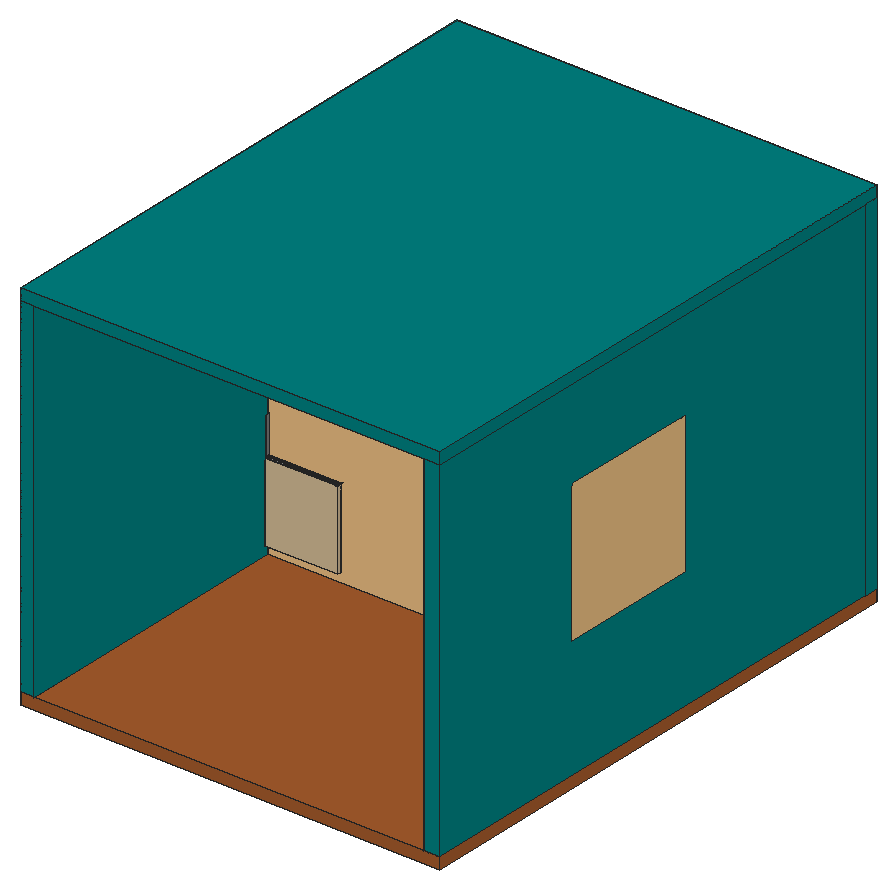
# SketchUp Ruby script. Lengths in inches.
U = 1.inch
M = Sketchup.active_model
def pt(a) = Geom::Point3d.new(a.map { |v| v * U })
def face(e, loops, mat)
  f = e.add_face(loops[0].map { |a| pt(a) })
  loops[1..].each { |l| e.add_face(l.map { |a| pt(a) }).erase! }
  f.material = f.back_material = mat if mat
  f
end
# faces: each face lists its corners as indices into pts; further lists are holes
def faces(e, pts, list, mat = nil) = list.each { |f| face(e, (f[0].is_a?(Array) ? f : [f]).map { |l| l.map { |i| pts[i] } }, mat) }
# xy, xz, yz: faces in a plane at the given z, y or x. An outline is a flat list of corners, or four numbers for a rectangle; further outlines are holes
def ring(l) = l.size == 4 ? [[l[0], l[1]], [l[2], l[1]], [l[2], l[3]], [l[0], l[3]]] : l.each_slice(2).to_a
def flat(e, list, mat, &to3) = list.each { |f| face(e, (f[0].is_a?(Array) ? f : [f]).map { |l| ring(l).map { |u, v| to3.(u, v) } }, mat) }
def xy(e, z, list, mat = nil) = flat(e, list, mat) { |x, y| [x, y, z] }
def xz(e, y, list, mat = nil) = flat(e, list, mat) { |x, z| [x, y, z] }
def yz(e, x, list, mat = nil) = flat(e, list, mat) { |y, z| [x, y, z] }
def lines(e, pts, list) = list.each { |a, b| e.add_line(pt(pts[a]), pt(pts[b])) }
# prism: a flat outline (further loops are holes) pulled along v
def prism(e, loops, v, mat = nil)
  f = face(e, loops, mat); d = Geom::Vector3d.new(v.map { |x| x * U })
  f.pushpull(f.normal.samedirection?(d) ? d.length : -d.length)
end
def box(e, o, s, mat = nil) = prism(e, [[o, [o[0] + s[0], o[1], o[2]], [o[0] + s[0], o[1] + s[1], o[2]], [o[0], o[1] + s[1], o[2]]]], [0, 0, s[2]], mat)
def at(x, y, z, deg = 0) = Geom::Transformation.translation(pt([x, y, z])) * Geom::Transformation.rotation(ORIGIN, Z_AXIS, deg.degrees)
def axes(o, x, y, z) = Geom::Transformation.new([*x, 0, *y, 0, *z, 0, *pt(o).to_a, 1])
def part(name) = M.definitions.add(name)
# library, detail: a bought-in or finely detailed component or shape, given as its bounding box
def library(name, o, s) = part(name).tap { |d| box(d.entities, o, s) }
def detail(e, o, s) = box(e.add_group.entities, o, s)
def put(e, d, t, mat = nil) = e.add_instance(d, t).tap { |i| i.material = mat if mat }
def group(e, t, mat = nil) = e.add_group.tap { |g| g.transformation = t; g.material = mat if mat }.entities
root = M.entities
M.materials.add("CLC2-PC-Blanc INTER").color = [249, 249, 249]
M.materials.add("Material \#1").color = [0, 0, 0]
M.materials.add("Standardmaterial30").color = [86, 86, 86]
M.materials.add("[0031_PapayaWhip]").color = [199, 195, 183]
M.materials.add("[0031_PapayaWhip]1").color = [211, 117, 3]
M.materials.add("[0079_Teal]").color = [0, 128, 128]
M.materials.add("[0088_Aquamarine]").color = [127, 255, 212]
M.materials.add("[0091_MintCream]").color = [201, 113, 3]
M.materials.add("[0099_LightSteelBlue]").color = [176, 196, 222]
M.materials.add("[Blacktop Old 01]").color = [132, 136, 139]
M.materials.add("[Blinds Wood White]").color = [138, 137, 139]
M.materials.add("[Encaustic Tile Circular 01]").color = [123, 123, 122]
M.materials.add("[Formica Beige]").color = [211, 187, 149]
M.materials.add("[Ornate Tile 01]").color = [202, 202, 202]
M.materials.add("[Resin Turquoise]").color = [117, 218, 223]
M.materials.add("[Stone Marble]").color = [143, 138, 136]
M.materials.add("[Stone Vein Gray]").color = [166, 165, 165]
M.materials.add("[Terrazzo Light Blue]").color = [196, 214, 227]
M.materials.add("[Tile Hexagon White]").color = [213, 206, 204]
M.materials.add("[Translucent Glass Gray]").color = [128, 128, 128]
M.materials["[Translucent Glass Gray]"].alpha = 0.5
M.materials.add("[Wood Board Cork]").color = [215, 201, 115]
M.materials.add("[Wood Cherry Original]").color = [152, 86, 42]
M.materials.add("[Wood Square Tile 01]").color = [164, 91, 44]
M.materials.add("utensils_wood_2").color = [89, 58, 24]
c1 = library("Group\#12",[-32.31,-359.75,0.0625],[113.14,110.83,100])
c2 = library("Group\#19",[-370.5625,-274.21,5.8125],[90.77,166.34,120.375])
c3 = library("Group\#17",[-278.11,-348.23,5.8],[187.87,187.87,121.65])
c4 = library("Group\#13",[-77.16,-243.45,0.06],[77.78,77.39,334.5])
c5 = library("Group\#11",[5.16,-238.13,0.06],[77.38,77.77,330.87])
c6 = library("Group\#21",[162.6875,-473.8,0.53],[157.34,166.37,329.78])
c7 = library("Group\#14",[-424.81,-54.29,0.29],[386.66,43.55,222.03])
c8 = library("Group\#20",[70.49,-356.56,0.0625],[143.03,166.7,314.72])
c9 = library("Group\#22",[-91.3125,-441.93,-0.01],[120,70.11,138.07])
c10 = library("Group\#16",[-375.96,-353.73,0.05],[297.45,297.44,31.27])
c11 = library("Group\#18",[-284.5,-166.25,5.875],[106.63,106.63,250.48])
c12 = part("Kitchen countertop accessories")
p = [[424.81,473.8,0.01],[425.81,473.8,0.01],[425.81,474.8,0.01]]
lines(c12.entities,p,[[0,1],[2,0]])
put(c12.entities,c1,at(424.81,473.8,0.01))
put(c12.entities,c2,at(424.81,473.8,0.01))
put(c12.entities,c3,at(424.81,473.8,0.01))
put(c12.entities,c4,at(424.81,473.8,0.01))
put(c12.entities,c5,at(424.81,473.8,0.01))
put(c12.entities,c6,at(424.81,473.8,0.01))
put(c12.entities,c7,at(424.81,473.8,0.01),"utensils_wood_2")
put(c12.entities,c8,at(424.81,473.8,0.01))
put(c12.entities,c9,at(424.81,473.8,0.01))
put(c12.entities,c10,at(424.81,473.8,0.01))
put(c12.entities,c11,at(424.81,473.8,0.01))
c13 = library("pellawindow\#4",[0,-3.05,0],[47.5,4.65,53.5])
c14 = library("007",[-28.95,-65.99,21.26],[5.48,1.13,0.69])
c15 = library("5-HOTTE ASPIRANTE CLC2",[-15.16,-17.72,-0.29],[30.34,17.72,30.09])
c16 = library("Hob1",[-15.52,-17.72,0],[31.04,35.44,3.4])
c17 = library("6-FOUR H60 CLC2",[0,-1.15,0],[23.5,21.54,23.5])
c18 = library("2-TABLE DE CUISSON CLC2",[-11.42,-10.04,0],[22.84,20.08,1.26])
c19 = part("CLC2-Ele02")
prism(c19.entities,[[[0.84,-0.32,0.16],[0.84,-0.33,0.02],[0.84,-0.34,-0.125],[0.84,-0.36,-0.27],[0.84,-0.39,-0.41],[0.84,-0.43,-0.55],[0.84,-0.47,-0.68],[0.84,-0.51,-0.82],[0.84,-0.2,-0.84],[0.84,-0.07,0.84],[0.84,-0.375,0.87],[0.84,-0.35,0.73],[0.84,-0.33,0.59],[0.84,-0.32,0.44],[0.84,-0.32,0.3]]],[-0.83,0,0],"CLC2-PC-Blanc INTER")
prism(c19.entities,[[[-0.01,-0.32,0.16],[-0.01,-0.33,0.02],[-0.01,-0.34,-0.125],[-0.01,-0.36,-0.27],[-0.01,-0.39,-0.41],[-0.01,-0.43,-0.55],[-0.01,-0.47,-0.68],[-0.01,-0.51,-0.82],[-0.01,-0.2,-0.84],[-0.01,-0.07,0.84],[-0.01,-0.375,0.87],[-0.01,-0.35,0.73],[-0.01,-0.33,0.59],[-0.01,-0.32,0.44],[-0.01,-0.32,0.3]]],[-0.83,0,0],"CLC2-PC-Blanc INTER")
xy(c19.entities,-1.57,[[-1.44,-0.19,1.44,0]],"CLC2-PC-Blanc INTER")
xy(c19.entities,-1.5,[[-1.375,-0.12,1.375,0]],"CLC2-PC-Blanc INTER")
xy(c19.entities,-0.87,[[-0.85,-0.29,0.85,-0.12]],"CLC2-PC-Blanc INTER")
xy(c19.entities,0.87,[[-0.85,-0.29,0.85,-0.12]],"CLC2-PC-Blanc INTER")
xy(c19.entities,1.5,[[-1.375,-0.12,1.375,0]],"CLC2-PC-Blanc INTER")
xy(c19.entities,1.57,[[-1.44,-0.19,1.44,0]],"CLC2-PC-Blanc INTER")
xz(c19.entities,-0.12,[[[-1.375,-1.5,-1.41,-1.3,-1.4375,-1.04,-1.46,-0.78,-1.48,-0.52,-1.5,0,-1.48,0.52,-1.46,0.78,-1.4375,1.04,-1.41,1.3,-1.375,1.5,1.375,1.5,1.41,1.3,1.4375,1.04,1.46,0.78,1.48,0.52,1.5,0,1.48,-0.52,1.46,-0.78,1.4375,-1.04,1.41,-1.3,1.375,-1.5],[-0.85,-0.87,0.85,0.87]]],"CLC2-PC-Blanc INTER")
xz(c19.entities,0,[[-1.44,-1.57,-1.48,-1.3125,-1.51,-1.05,-1.54,-0.79,-1.56,-0.53,-1.57,-0.26,-1.57,0.26,-1.56,0.53,-1.54,0.79,-1.51,1.05,-1.48,1.3125,-1.44,1.57,0,1.57,0,1.5,-1.375,1.5,-1.41,1.3,-1.4375,1.04,-1.46,0.78,-1.48,0.52,-1.5,0,-1.48,-0.52,-1.46,-0.78,-1.4375,-1.04,-1.41,-1.3,-1.375,-1.5,0,-1.5,0,-1.57],[0,-1.57,0,-1.5,1.375,-1.5,1.41,-1.3,1.4375,-1.04,1.46,-0.78,1.48,-0.52,1.5,0,1.48,0.52,1.46,0.78,1.4375,1.04,1.41,1.3,1.375,1.5,0,1.5,0,1.57,1.44,1.57,1.48,1.3125,1.51,1.05,1.54,0.79,1.56,0.53,1.57,0.26,1.57,-0.26,1.56,-0.53,1.54,-0.79,1.51,-1.05,1.48,-1.3125,1.44,-1.57]],"CLC2-PC-Blanc INTER")
yz(c19.entities,-1.57,[[-0.0625,-0.26,-0.06,0,0,0,0,-0.26],[-0.06,0,-0.0625,0.26,0,0.26,0,0]],"CLC2-PC-Blanc INTER")
yz(c19.entities,-0.85,[[-0.29,-0.87,-0.12,-0.87,-0.12,0.87,-0.29,0.87,-0.29,0.79,-0.3125,0.53,-0.32,0.26,-0.33,0,-0.32,-0.26,-0.3125,-0.53,-0.29,-0.79]],"CLC2-PC-Blanc INTER")
yz(c19.entities,0.85,[[-0.29,-0.87,-0.29,-0.79,-0.3125,-0.53,-0.32,-0.26,-0.33,0,-0.32,0.26,-0.3125,0.53,-0.29,0.79,-0.29,0.87,-0.12,0.87,-0.12,-0.87]],"CLC2-PC-Blanc INTER")
yz(c19.entities,1.57,[[-0.0625,-0.26,0,-0.26,0,0,-0.06,0],[-0.06,0,0,0,0,0.26,-0.0625,0.26]],"CLC2-PC-Blanc INTER")
p = [[-1.32,-0.3125,0.53],[-1.34,-0.29,0.79],[-1.37,-0.27,1.05],[-1.4,-0.23,1.3125],[-1.44,-0.19,1.57],[-1.48,-0.15,1.3125],
  [-1.51,-0.12,1.05],[-1.54,-0.09,0.79],[-1.56,-0.07,0.53],[-1.57,-0.0625,0.26],[-1.57,-0.06,0],[-1.57,-0.0625,-0.26],
  [-1.56,-0.07,-0.53],[-1.54,-0.09,-0.79],[-1.51,-0.12,-1.05],[-1.48,-0.15,-1.3125],[-1.44,-0.19,-1.57],[-1.4,-0.23,-1.3125],
  [-1.37,-0.27,-1.05],[-1.34,-0.29,-0.79],[-1.32,-0.3125,-0.53],[-1.31,-0.32,-0.26],[-1.3,-0.33,0],[-1.31,-0.32,0.26],
  [1.34,-0.29,0.79],[1.32,-0.3125,0.53],[1.31,-0.32,0.26],[1.3,-0.33,0],[1.31,-0.32,-0.26],[1.32,-0.3125,-0.53],
  [1.34,-0.29,-0.79],[1.37,-0.27,-1.05],[1.4,-0.23,-1.3125],[1.44,-0.19,-1.57],[1.48,-0.15,-1.3125],[1.51,-0.12,-1.05],
  [1.54,-0.09,-0.79],[1.56,-0.07,-0.53],[1.57,-0.0625,-0.26],[1.57,-0.06,0],[1.57,-0.0625,0.26],[1.56,-0.07,0.53],
  [1.54,-0.09,0.79],[1.51,-0.12,1.05],[1.48,-0.15,1.3125],[1.44,-0.19,1.57],[1.4,-0.23,1.3125],[1.37,-0.27,1.05],
  [-1.44,0,-1.57],[-1.48,0,-1.3125],[1.44,0,-1.57],[1.48,0,-1.3125],[-1.375,0,-1.5],[-1.41,0,-1.3],
  [-1.41,-0.12,-1.3],[-1.375,-0.12,-1.5],[1.41,0,-1.3],[1.375,0,-1.5],[1.375,-0.12,-1.5],[1.41,-0.12,-1.3],
  [-1.51,0,-1.05],[1.51,0,-1.05],[-1.4375,0,-1.04],[-1.4375,-0.12,-1.04],[1.4375,0,-1.04],[1.4375,-0.12,-1.04],
  [0.85,-0.29,-0.87],[-0.85,-0.29,-0.87],[-0.85,-0.29,-0.79],[-1.33,-0.29,-0.79],[1.33,-0.29,-0.79],[0.85,-0.29,-0.79],
  [-1.54,0,-0.79],[1.54,0,-0.79],[-1.46,0,-0.78],[-1.46,-0.12,-0.78],[1.46,0,-0.78],[1.46,-0.12,-0.78],
  [-0.85,-0.3125,-0.53],[0.85,-0.3125,-0.53],[-1.56,0,-0.53],[-1.48,0,-0.52],[-1.48,-0.12,-0.52],[1.48,0,-0.52],
  [1.48,-0.12,-0.52],[1.56,0,-0.53],[-0.85,-0.32,-0.26],[0.85,-0.32,-0.26],[-1.57,0,-0.26],[-1.49,0,-0.26],
  [-1.49,-0.12,-0.26],[1.49,0,-0.26],[1.49,-0.12,-0.26],[1.57,0,-0.26],[-0.85,-0.33,0],[0.85,-0.33,0],
  [-1.5,0,0],[-1.5,-0.12,0],[1.5,0,0],[1.5,-0.12,0],[-0.85,-0.32,0.26],[0.85,-0.32,0.26],
  [-1.49,0,0.26],[-1.49,-0.12,0.26],[1.49,0,0.26],[1.49,-0.12,0.26],[-0.85,-0.3125,0.53],[0.85,-0.3125,0.53],
  [-1.57,0,0.26],[-1.56,0,0.53],[-1.48,0,0.52],[-1.48,-0.12,0.52],[1.48,0,0.52],[1.48,-0.12,0.52],
  [1.57,0,0.26],[1.56,0,0.53],[-0.85,-0.29,0.79],[-1.33,-0.29,0.79],[1.33,-0.29,0.79],[0.85,-0.29,0.79],
  [-1.54,0,0.79],[-1.46,0,0.78],[-1.46,-0.12,0.78],[1.46,0,0.78],[1.46,-0.12,0.78],[1.54,0,0.79],
  [-0.85,-0.29,0.87],[0.85,-0.29,0.87],[-1.4375,0,1.04],[-1.4375,-0.12,1.04],[-1.51,0,1.05],[1.4375,0,1.04],
  [1.4375,-0.12,1.04],[1.51,0,1.05],[-1.41,0,1.3],[-1.41,-0.12,1.3],[1.41,0,1.3],[1.41,-0.12,1.3],
  [-1.48,0,1.3125],[1.48,0,1.3125],[-1.44,0,1.57],[1.44,0,1.57],[-1.375,0,1.5],[-1.375,-0.12,1.5],
  [1.375,0,1.5],[1.375,-0.12,1.5]]
faces(c19.entities,p,[[0,1,2,3,4,5,6,7,8,9,10,11,12,13,14,15,16,17,18,19,20,21,22,23],[24,25,26,27,28,29,30,31,32,33,34,35,36,37,38,39,40,41,42,43,44,45,46,47],[48,16,15,49],[32,17,16,33],[33,50,51,34],[52,53,54,55],[56,57,58,59],[31,18,17,32],
  [49,15,14,60],[34,51,61,35],[53,62,63,54],[64,56,59,65],[66,67,68,69,19,18,31,30,70,71],[60,14,13,72],[35,61,73,36],[62,74,75,63],
  [76,64,65,77],[69,68,78,20,19],[71,70,30,29,79],[72,13,12,80],[74,81,82,75],[83,76,77,84],[36,73,85,37],[20,78,86,21],
  [79,29,28,87],[80,12,11,88],[81,89,90,82],[91,83,84,92],[37,85,93,38],[21,86,94,22],[87,28,27,95],[89,96,97,90],
  [98,91,92,99],[22,94,100,23],[95,27,26,101],[96,102,103,97],[104,98,99,105],[23,100,106,0],[101,26,25,107],[108,9,8,109],
  [102,110,111,103],[112,104,105,113],[40,114,115,41],[0,106,116,117,1],[107,25,24,118,119],[109,8,7,120],[110,121,122,111],[123,112,113,124],
  [41,115,125,42],[116,126,127,119,118,24,47,2,1,117],[121,128,129,122],[120,7,6,130],[131,123,124,132],[42,125,133,43],[128,134,135,129],[136,131,132,137],
  [46,3,2,47],[130,6,5,138],[43,133,139,44],[138,5,4,140],[4,3,46,45],[44,139,141,45],[134,142,143,135],[144,136,137,145]],"CLC2-PC-Blanc INTER")
c20 = part("2-PRISEELC CLC2")
put(c20.entities,c19,axes([0,0,0],[1,0,0],[0,0,-1],[0,1,0]))
c21 = library("15-PRODUITS CUISINE CLC2",[-1.94,-2.15,0],[3.93,3.94,5.51])
c22 = library("12-PRODUITS CUISINE CLC2",[-1.08,-1.08,0],[2.16,2.16,5.375])
c23 = library("15-PRODUITS CUISINE CLC2\#1",[-1.94,-2.15,0],[3.93,3.94,5.51])
c24 = library("Sink with drainboard",[-0.15,-0.12,-6.4],[37.85,20.23,20.6])
c25 = library("AS-120-mm",[0,0,0],[48,4.72,48])
c26 = library("9-POIGNEE CLC2",[-3.01,-0.26,0],[6.02,0.52,1.49])
c27 = library("2-POIGNEE CLC2",[-2.66,-0.49,0],[5.32,0.98,1.3])
c28 = library("Group\#4",[0,32.625,0],[131,82,57])
c29 = part("Union")
xy(c29.entities,0,[[0,51.67,0.1,82.93]],"[Tile Hexagon White]")
xy(c29.entities,0.04,[[0.1875,0,0,51.67,0.1,51.67,0.29,0]],"[Tile Hexagon White]")
xy(c29.entities,12.44,[[0.1875,0,0.29,0,0.1,51.67,0,51.67]],"[Tile Hexagon White]")
xy(c29.entities,29.375,[[0,51.67,0.1,82.93]],"[Tile Hexagon White]")
xz(c29.entities,0,[[0.1875,0.04,0.29,12.44]],"[Tile Hexagon White]")
xz(c29.entities,51.67,[[0,0,0.1,0.04],[0,12.44,0.1,29.375]],"[Tile Hexagon White]")
xz(c29.entities,82.93,[[0,0,0.1,29.375]],"[Tile Hexagon White]")
yz(c29.entities,0,[[51.67,0,82.93,29.375]],"[Tile Hexagon White]")
yz(c29.entities,0.1,[[51.67,0,82.93,29.375]],"[Encaustic Tile Circular 01]")
p = [[0,51.67,0.04],[0.1875,0,0.04],[0.1875,0,12.44],[0,51.67,12.44],[0.29,0,0.04],[0.1,51.67,0.04],
  [0.1,51.67,12.44],[0.29,0,12.44]]
faces(c29.entities,p,[[0,1,2,3]],"[Tile Hexagon White]")
faces(c29.entities,p,[[4,5,6,7]],"[Encaustic Tile Circular 01]")
c30 = part("Group\#39")
box(c30.entities,[0,-0.16,0],[14.04,0.16,8.44])
c31 = library("Group\#36",[0,0,0],[13.37,2.97,7.55])
c32 = part("Union\#1")
xy(c32.entities,0,[[0,48.27,0.1,124.86]])
xy(c32.entities,0,[[0,0,0.1,48.27]],"[Encaustic Tile Circular 01]")
xy(c32.entities,10.36,[[0,0,0.1,47.52]],"[Encaustic Tile Circular 01]")
xy(c32.entities,29.13,[[0,47.52,0.1,124.86]])
xz(c32.entities,0,[[0,0,0.1,10.36]],"[Encaustic Tile Circular 01]")
xz(c32.entities,47.52,[[0,10.36,0.1,29.13]])
xz(c32.entities,124.86,[[0,0,0.1,29.13]])
yz(c32.entities,0,[[0,0,0,10.36,47.52,10.36,47.52,29.13,124.86,29.13,124.86,0]],"[Encaustic Tile Circular 01]")
yz(c32.entities,0.1,[[48.27,0,124.86,0,124.86,29.13,47.52,29.13,47.52,10.36,48.27,10.36]])
yz(c32.entities,0.1,[[0,0,48.27,10.36]],"[Encaustic Tile Circular 01]")
c33 = library("Group\#182",[0,0,0],[42.16,31.84,40.44])
c34 = library("Group\#184",[0,0,-7.25],[98.84,110.93,7.25])
xz(root,161.23,[[99.375,31.2,126.76,31.21]],"[Stone Vein Gray]")
xz(root,176.99,[[99.375,31.2,126.76,31.21]],"[Stone Vein Gray]")
yz(root,99.375,[[161.23,31.2,176.99,31.21]],"[Stone Vein Gray]")
p = [[29.43,157.1875,3],[29.43,157.1875,30],[126.76,161.23,31.2],[126.76,176.99,31.2],[0,18.6875,120],[0,186.6875,120],
  [143.41,186.6875,120],[143.41,18.6875,120]]
lines(root,p,[[0,1],[2,3],[4,5],[5,6],[6,7],[7,4]])
put(root,c12,axes([19.84,158.83,30.625],[0,0.0275,0],[-0.0275,0,0],[0,0,0.0275]))
put(root,c13,at(1.5,102.92,42.625,90))
put(root,c14,axes([77.75,192.75,48.53],[0,0,0.87],[0,0.5481,0],[-0.87,0,0]))
put(root,c14,axes([71.76,192.75,48.53],[0,0,0.87],[0,0.5481,0],[-0.87,0,0]))
put(root,c14,axes([53.76,192.74,48.77],[0,0,0.87],[0,0.5481,0],[-0.87,0,0]))
put(root,c14,axes([95.6,192.75,52.97],[0,0,0.87],[0,0.5481,0],[-0.87,0,0]))
put(root,c14,axes([113.81,192.75,48.53],[0,0,0.87],[0,0.5481,0],[-0.87,0,0]))
put(root,c14,axes([141.37,192.75,48.53],[0,0,0.87],[0,0.5481,0],[-0.87,0,0]))
put(root,c14,axes([143.24,192.75,48.53],[0,0,0.87],[0,0.5481,0],[-0.87,0,0]))
put(root,c14,axes([-6.01,115.6,38.68],[0,-0.87,0],[-0.5481,0,0],[0,0,-0.87]))
put(root,c14,axes([-6.05,129.48,46.95],[0,0,0.87],[-0.5481,0,0],[0,-0.87,0]))
put(root,c14,axes([-6.05,132.24,46.95],[0,0,0.87],[-0.5481,0,0],[0,-0.87,0]))
put(root,c14,axes([-6.05,115.6,44.93],[0,-0.87,0],[-0.5481,0,0],[0,0,-0.87]))
put(root,c14,axes([-5.95,115.6,33.24],[0,-0.87,0],[-0.5481,0,0],[0,0,-0.87]))
put(root,c15,axes([6.52,134.6875,76.78],[0.00015,0.99911,0.01208],[-0.99993,0,0.01209],[0.01595,-0.01595,1.31981]))
put(root,c16,axes([16.75,138.99,30.625],[0.68089,0,0],[0,0.79341,0],[0,0,1.1662]),"Material \#1")
put(root,c17,axes([51.02,159.49,30.625],[1,0,0],[0,1,0],[0,0,1.05]))
put(root,c18,at(16.86,138.26,30.625))
put(root,c20,axes([18.77,181.49,47.7],[1,0,0],[0,0,1],[0,-1,0]))
put(root,c21,axes([75.13,173.46,72.5],[1.17,0,0],[0,1.17,0],[0,0,1.07359]))
put(root,c22,axes([85.96,170.82,72.5],[1.17,0,0],[0,1.17,0],[0,0,1.07359]))
put(root,c23,axes([79.76,173.46,72.5],[1.17,0,0],[0,1.17,0],[0,0,1.07359]))
put(root,c22,axes([83.6,173.46,72.5],[1.17,0,0],[0,1.17,0],[0,0,1.07359]))
put(root,c24,axes([96.12,161.06,31.38],[1,0,0],[0,1,-0.00308],[0,0.00308,1]))
put(root,c25,at(143.41,56.625,41.24,90))
put(root,c26,axes([18.44,167.1875,73.7],[1,0,0],[0,0,0.99928],[0,-1.00073,0]))
put(root,c26,axes([18.44,167.1875,61.05],[1,0,0],[0,0,0.99928],[0,-1.00073,0]))
put(root,c26,axes([122.88,167.1875,73.7],[1,0,0],[0,0,0.99928],[0,-1.00073,0]))
put(root,c26,axes([122.88,167.1875,61.05],[1,0,0],[0,0,0.99928],[0,-1.00073,0]))
put(root,c27,axes([37.15,167.1875,73.34],[0,0,1],[-1,0,0],[0,-1,0]))
put(root,c27,axes([91.29,167.1875,73.34],[0,0,1],[-1,0,0],[0,-1,0]))
put(root,c28,at(4.5,67.5625,0),"[Terrazzo Light Blue]")
g1 = group(root,at(4.5,182.1875,60),"[Wood Board Cork]")
xy(g1,0,[[1,-14,49.09,0],[85.16,-14,133,0]],"[Wood Board Cork]")
xy(g1,11.5,[[49.09,-14,85.16,0]],"[Wood Board Cork]")
xy(g1,12.5,[[50.09,-14,84.16,-0.75]],"[0031_PapayaWhip]")
xy(g1,22.94,[[50.09,-14,84.16,-0.75]],"[0031_PapayaWhip]")
xy(g1,23.94,[[1,-14,49.09,0],[49.09,-14,85.16,0],[85.16,-14,133,0]],"[Wood Board Cork]")
xz(g1,-14,[[1,0,49.09,23.94],[85.16,0,133,23.94],[[49.09,11.5,85.16,23.94],[50.09,12.5,84.16,22.94]]],"[0031_PapayaWhip]")
xz(g1,-0.75,[[50.09,12.5,84.16,22.94]],"[0031_PapayaWhip]")
xz(g1,0,[[1,0,1,23.94,133,23.94,133,0,85.16,0,85.16,11.5,49.09,11.5,49.09,0]],"[0031_PapayaWhip]")
yz(g1,1,[[-14,0,0,23.94]],"[0031_PapayaWhip]")
yz(g1,49.09,[[-14,0,0,11.5]],"[Wood Board Cork]")
yz(g1,84.16,[[-14,12.5,-0.75,22.94]],"[0031_PapayaWhip]")
yz(g1,85.16,[[-14,0,0,11.5]],"[Wood Board Cork]")
yz(g1,133,[[-14,0,0,23.94]],"[0031_PapayaWhip]")
g2 = group(g1,at(50.09,-14,12.5))
yz(g2,0,[[0,0,13.25,10.44]])
g3 = group(root,at(4.5,168.1875,60),"[Blinds Wood White]")
box(g3,[31.16,-1,0],[17.93,1,23.94],"[0031_PapayaWhip]")
xy(g3,0,[[85.16,-1,103,0]],"[0031_PapayaWhip]")
xy(g3,23.94,[[85.16,-1,103,0]],"[0031_PapayaWhip]")
xz(g3,-1,[[85.16,0,103,23.94]],"[0031_PapayaWhip]")
xz(g3,0,[[85.16,0,103,23.94]],"[0031_PapayaWhip]")
yz(g3,85.16,[[-1,0,0,23.94]],"[0031_PapayaWhip]")
yz(g3,103,[[-1,0,0,23.94]],"[0031_PapayaWhip]")
p = [[84,-0.34,22.94],[84,-0.54,22.94]]
lines(g3,p,[[0,1]])
g4 = group(g3,at(0,-1,0),"[Wood Board Cork]")
xy(g4,0,[[0,0,1,15],[1,0,31,1]],"[Wood Board Cork]")
xy(g4,11.89,[[1,0,31,1]],"[Wood Board Cork]")
xy(g4,12.05,[[1,0,31,1]],"[0091_MintCream]")
xy(g4,23.94,[[0,0,1,15],[1,0,31,1]],"[Wood Board Cork]")
xz(g4,0,[[0,0,1,23.94],[1,0,31,11.89],[1,12.05,31,23.94]],"[Wood Board Cork]")
xz(g4,1,[[1,0,31,11.89],[1,11.89,31,12.05],[1,12.05,31,23.94]],"[0091_MintCream]")
xz(g4,15,[[0,0,1,23.94]],"[0091_MintCream]")
yz(g4,0,[[0,0,15,23.94]],"[0091_MintCream]")
yz(g4,1,[[0,0,1,11.89],[1,0,15,23.94],[0,11.89,1,12.05],[0,12.05,1,23.94]],"[0091_MintCream]")
yz(g4,31,[[0,0,1,11.89],[0,12.05,1,23.94]],"[Wood Board Cork]")
g5 = group(g3,at(103.16,-1,12.05),"[Wood Board Cork]")
xy(g5,0,[[0,0,29.84,1]],"[0031_PapayaWhip]1")
xy(g5,11.89,[[0,0,29.84,1]],"[Wood Board Cork]")
xz(g5,0,[[0,0,29.84,11.89]],"[Wood Board Cork]")
xz(g5,1,[[0,0,29.84,11.89]],"[0031_PapayaWhip]1")
yz(g5,0,[[0,0,1,11.89]],"[Wood Board Cork]")
yz(g5,29.84,[[0,0,1,11.89]],"[Wood Board Cork]")
g6 = group(g3,at(103.16,-1,0),"[Wood Board Cork]")
xy(g6,0,[[0,0,29.84,1]],"[Wood Board Cork]")
xy(g6,11.89,[[0,0,29.84,1]],"[Wood Board Cork]")
xz(g6,0,[[0,0,29.84,11.89]],"[Wood Board Cork]")
xz(g6,1,[[0,0,29.84,11.89]],"[Wood Cherry Original]")
yz(g6,0,[[0,0,1,11.89]],"[Wood Cherry Original]")
yz(g6,29.84,[[0,0,1,11.89]],"[Wood Board Cork]")
g7 = group(g3,at(133.16,-1,0),"[Wood Board Cork]")
xy(g7,0,[[0,0,2.25,15]],"[Wood Board Cork]")
xy(g7,23.94,[[0,0,2.25,15]],"[Wood Board Cork]")
xz(g7,0,[[0,0,2.25,23.94]],"[Wood Board Cork]")
xz(g7,15,[[0,0,2.25,23.94]],"[Wood Cherry Original]")
yz(g7,0,[[0,0,1,23.94],[1,0,15,23.94]],"[Wood Cherry Original]")
yz(g7,2.25,[[0,0,15,23.94]],"[Wood Board Cork]")
g8 = group(root,at(54.59,168.1875,72.5))
box(g8,[-1,0,0],[1,13.25,10.44])
g9 = group(root,at(28.5,67.5625,3),"[Formica Beige]")
box(g9,[0,56.625,0],[1,29.84,13.54])
box(g9,[0,56.625,20.35],[1,29.84,6.65])
box(g9,[0,56.625,13.62],[1,29.84,6.65])
xy(g9,0,[[0,32.625,1,44.42],[0,44.58,1,56.47]])
xy(g9,0,[[-24,31.5,1,32.47]],"[Terrazzo Light Blue]")
xy(g9,26.1,[[0.125,32.72,1,44.32],[0.125,44.68,1,56.37]],"Standardmaterial30")
xy(g9,26.78,[[0.5625,32.72,1,44.32],[0.57,44.68,1,56.37]],"Standardmaterial30")
xy(g9,26.9,[[0.125,32.72,0.5625,44.32],[0.125,44.68,0.57,56.37]])
xy(g9,27,[[0,32.625,1,44.42],[0,44.58,1,56.47]])
xy(g9,27,[[-24,31.5,1,32.47]],"[Terrazzo Light Blue]")
xz(g9,31.5,[[-24,0,1,27]],"[Formica Beige]")
xz(g9,32.47,[[-24,0,1,27]],"[Terrazzo Light Blue]")
xz(g9,32.625,[[0,0,1,27]])
xz(g9,32.72,[[0.125,26.1,0.125,26.9,0.5625,26.9,0.5625,26.78,1,26.78,1,26.1]],"Standardmaterial30")
xz(g9,44.32,[[0.125,26.1,1,26.1,1,26.78,0.5625,26.78,0.5625,26.9,0.125,26.9]],"Standardmaterial30")
xz(g9,44.42,[[0,0,1,27]])
xz(g9,44.58,[[0,0,1,27]])
xz(g9,44.68,[[0.125,26.1,0.125,26.9,0.57,26.9,0.57,26.78,1,26.78,1,26.1]],"Standardmaterial30")
xz(g9,56.37,[[0.125,26.1,1,26.1,1,26.78,0.57,26.78,0.57,26.9,0.125,26.9]],"Standardmaterial30")
xz(g9,56.47,[[0,0,1,27]])
yz(g9,-24,[[31.5,0,32.47,27]],"[Terrazzo Light Blue]")
yz(g9,0,[[32.625,0,44.42,27],[44.42,0,44.58,27],[44.58,0,56.47,27]])
yz(g9,0.125,[[32.72,26.1,44.32,26.9],[44.68,26.1,56.37,26.9]],"Standardmaterial30")
yz(g9,0.5625,[[32.72,26.78,44.32,26.9]])
yz(g9,0.57,[[44.68,26.78,56.37,26.9]])
yz(g9,1,[[[32.625,26,44.42,27],[32.72,26.1,44.32,26.78]],[[44.58,26,56.47,27],[44.68,26.1,56.37,26.78]]])
yz(g9,1,[[31.5,0,32.47,27],[32.625,0,44.42,26],[44.58,0,56.47,26]],"[Formica Beige]")
g10 = group(g9,at(0,86.625,0))
prism(g10,[[[1,3,0],[1,0,0],[0,0,0],[0,4,0],[1,4,0]]],[0,0,27])
g11 = group(root,at(29.5,157.1875,3),"[Stone Marble]")
xy(g11,0,[[22.16,0,28,1],[28.16,0,46,1],[64.16,0,82,1],[82.16,0,94,1],[94.16,0,106,1],
  [106.16,0,108.22,25]])
xy(g11,0,[[4.16,0,22,1]],"[Terrazzo Light Blue]")
xy(g11,27,[[22.16,0,28,1],[28.16,0,46,1],[64.16,0,82,1],[82.16,0,94,1],[94.16,0,106,1]])
xy(g11,27,[[4.16,0,22,1],[106.16,0,108.22,25]],"[Terrazzo Light Blue]")
xz(g11,0,[[4.16,0,22,27],[22.16,0,28,27],[28.16,0,46,27],[64.16,0,82,27],[82.16,0,94,27],
  [94.16,0,106,27],[106.16,0,108.22,27]],"[Formica Beige]")
xz(g11,1,[[22.16,0,28,27],[28.16,0,46,27],[64.16,0,82,27],[82.16,0,94,27],[94.16,0,106,27]])
xz(g11,1,[[4.16,0,22,27]],"[Terrazzo Light Blue]")
xz(g11,25,[[106.16,0,108.22,27]])
yz(g11,4.16,[[0,0,1,27]],"[Terrazzo Light Blue]")
yz(g11,22,[[0,0,1,27]],"[Terrazzo Light Blue]")
yz(g11,22.16,[[0,0,1,27]])
yz(g11,28,[[0,0,1,27]])
yz(g11,28.16,[[0,0,1,27]])
yz(g11,46,[[0,0,1,27]])
yz(g11,64.16,[[0,0,1,27]])
yz(g11,82,[[0,0,1,27]])
yz(g11,82.16,[[0,0,1,27]])
yz(g11,94,[[0,0,1,27]])
yz(g11,94.16,[[0,0,1,27]])
yz(g11,106,[[0,0,1,27]])
yz(g11,106.16,[[0,0,1,27],[1,0,25,27]])
yz(g11,108.22,[[0,0,25,27]],"[Formica Beige]")
g12 = group(g11,at(0,0,0),"[Formica Beige]")
box(g12,[0,0,0],[4,1,27])
g13 = group(root,at(75.5,158.1875,3),"[Formica Beige]")
prism(g13,[[[18.16,0,53.0625],[18.16,0,27],[18.16,0,0],[0,0,0],[0,0,27],[0,0,53.0625]]],[0,-1,0])
g14 = group(root,at(4.5,100.1875,30))
xy(g14,-0.22,[[0,-0.76,0,-0.72,24.6,-0.72,24.64,-0.76],[24.64,-0.76,24.6,-0.72,24.6,57.4,24.64,57.36],[0,-0.72,0,82,71,82,71,57.4,24.6,57.4,24.6,-0.72],[24.64,57.36,24.6,57.4,71,57.4,71,57.36]],"[Stone Vein Gray]")
xy(g14,0.625,[[0,-0.83,24.71,-0.83,24.67,-0.79,0,-0.79],[24.71,-0.83,24.71,57.29,24.67,57.33,24.67,-0.79],[0,-0.79,24.67,-0.79,24.67,57.33,71,57.33,71,82,0,82],[24.71,57.29,71,57.29,71,57.33,24.67,57.33]],"[Stone Vein Gray]")
xz(g14,-1.125,[[0,0,25,0.39]],"[Stone Vein Gray]")
xz(g14,57,[[25,0,71,0.39]],"[Stone Vein Gray]")
xz(g14,82,[[0,-0.22,71,0.625]],"[Stone Vein Gray]")
yz(g14,0,[[-0.76,-0.22,-0.92,-0.18,-0.95,-0.16,-0.99,-0.14,-1.02,-0.12,-1.05,-0.09,-1.08,-0.0625,-1.1,-0.03,-1.125,0,-1.125,0.39,-1.11,0.42,-1.05,0.51,-1,0.56,-0.97,0.58,-0.93,0.6,-0.87,0.62,-0.83,0.625,82,0.625,82,-0.22]],"[Stone Vein Gray]")
yz(g14,25,[[-1.125,0,57,0.39]],"[Stone Vein Gray]")
yz(g14,71,[[57.36,-0.22,82,-0.22,82,0.625,57.29,0.625,57.26,0.62,57.22,0.61,57.19,0.6,57.1,0.54,57.07,0.51,57.01,0.42,57,0.39,57,0,57.02,-0.03,57.05,-0.0625,57.08,-0.09,57.11,-0.12,57.17,-0.16,57.21,-0.18,57.24,-0.19]],"[Stone Vein Gray]")
p = [[0,-0.95,-0.16],[0,-0.92,-0.18],[24.79,-0.92,-0.18],[24.83,-0.95,-0.16],[0,-0.99,-0.14],[24.86,-0.99,-0.14],
  [24.79,57.21,-0.18],[24.83,57.17,-0.16],[24.86,57.14,-0.14],[0,-0.88,-0.19],[0,-0.84,-0.2],[24.72,-0.84,-0.2],
  [24.76,-0.88,-0.19],[24.72,57.28,-0.2],[24.76,57.24,-0.19],[0,-0.8,-0.21],[0,-0.76,-0.22],[24.64,-0.76,-0.22],
  [24.68,-0.8,-0.21],[24.64,57.36,-0.22],[24.68,57.32,-0.21],[71,57.17,-0.16],[71,57.14,-0.14],[71,57.28,-0.2],
  [71,57.24,-0.19],[71,57.21,-0.18],[71,57.36,-0.22],[71,57.32,-0.21],[0,-1.08,-0.0625],[0,-1.05,-0.09],
  [24.92,-1.05,-0.09],[24.95,-1.08,-0.0625],[0,-1.1,-0.03],[24.98,-1.1,-0.03],[24.92,57.08,-0.09],[24.95,57.05,-0.0625],
  [24.98,57.02,-0.03],[0,-1.02,-0.12],[24.89,-1.02,-0.12],[24.89,57.11,-0.12],[71,57.08,-0.09],[71,57.05,-0.0625],
  [71,57.02,-0.03],[71,57.11,-0.12],[0,-1.125,0],[25,-1.125,0],[25,57,0],[71,57,0],
  [0,-1.11,0.42],[0,-1.125,0.39],[25,-1.125,0.39],[24.99,-1.11,0.42],[0,-1.09,0.45],[24.97,-1.09,0.45],
  [25,57,0.39],[24.99,57.01,0.42],[24.97,57.03,0.45],[71,57,0.39],[71,57.01,0.42],[71,57.03,0.45],
  [0,-1.07,0.48],[24.95,-1.07,0.48],[0,-1.05,0.51],[24.93,-1.05,0.51],[0,-1.02,0.54],[24.9,-1.02,0.54],
  [24.95,57.05,0.48],[24.93,57.07,0.51],[24.9,57.1,0.54],[0,-1,0.56],[24.87,-1,0.56],[24.87,57.13,0.56],
  [71,57.05,0.48],[71,57.07,0.51],[71,57.1,0.54],[71,57.13,0.56],[0,-0.97,0.58],[24.84,-0.97,0.58],
  [0,-0.93,0.6],[24.81,-0.93,0.6],[24.84,57.16,0.58],[24.81,57.19,0.6],[0,-0.9,0.61],[24.78,-0.9,0.61],
  [0,-0.87,0.62],[24.74,-0.87,0.62],[0,-0.83,0.625],[24.71,-0.83,0.625],[24.78,57.22,0.61],[24.74,57.26,0.62],
  [24.71,57.29,0.625],[71,57.16,0.58],[71,57.22,0.61],[71,57.26,0.62],[71,57.19,0.6],[71,57.29,0.625],
  [71,82,0],[89.16,82,0],[89.16,58,0]]
faces(g14,p,[[0,1,2,3],[4,0,3,5],[3,2,6,7],[5,3,7,8],[9,10,11,12],[1,9,12,2],[12,11,13,14],[2,12,14,6],
  [15,16,17,18],[10,15,18,11],[18,17,19,20],[11,18,20,13],[8,7,21,22],[14,13,23,24],[6,14,24,25],[7,6,25,21],
  [20,19,26,27],[13,20,27,23],[28,29,30,31],[32,28,31,33],[31,30,34,35],[33,31,35,36],[37,4,5,38],[29,37,38,30],
  [38,5,8,39],[30,38,39,34],[35,34,40,41],[36,35,41,42],[39,8,22,43],[34,39,43,40],[44,32,33,45],[45,33,36,46],
  [46,36,42,47],[48,49,50,51],[52,48,51,53],[51,50,54,55],[53,51,55,56],[55,54,57,58],[56,55,58,59],[60,52,53,61],
  [62,60,61,63],[64,62,63,65],[61,53,56,66],[63,61,66,67],[65,63,67,68],[69,64,65,70],[70,65,68,71],[66,56,59,72],
  [67,66,72,73],[68,67,73,74],[71,68,74,75],[76,69,70,77],[78,76,77,79],[77,70,71,80],[79,77,80,81],[82,78,79,83],
  [84,82,83,85],[86,84,85,87],[85,83,88,89],[87,85,89,90],[83,79,81,88],[80,71,75,91],[89,88,92,93],[81,80,91,94],
  [88,81,94,92],[90,89,93,95]],"[Stone Vein Gray]")
lines(g14,p,[[96,97],[98,97]])
put(root,c29,at(4.5,99.25,30.625))
g15 = group(root,at(0,-53.3125,0),"[0088_Aquamarine]")
xy(g15,0,[[0,53.3125,0,240,143.41,240,143.41,235.5,4.5,235.5,4.5,53.3125]],"[0079_Teal]")
xy(g15,42.625,[[0,156.24,4.5,204.24]],"[0079_Teal]")
xy(g15,93.8125,[[0,156.24,4.5,204.24]],"[0079_Teal]")
xy(g15,120,[[0,53.3125,4.5,53.3125,4.5,235.5,143.41,235.5,143.41,240,0,240]],"[0079_Teal]")
xz(g15,53.3125,[[0,0,4.5,120]],"[0079_Teal]")
xz(g15,156.24,[[0,42.625,4.5,93.8125]],"[0079_Teal]")
xz(g15,204.24,[[0,42.625,4.5,93.8125]],"[0079_Teal]")
xz(g15,235.5,[[4.5,0,143.41,120]],"[0079_Teal]")
xz(g15,240,[[0,0,143.41,120]],"[0079_Teal]")
yz(g15,0,[[[53.3125,0,240,120],[156.24,42.625,204.24,93.8125]]],"[0079_Teal]")
yz(g15,4.5,[[[53.3125,0,235.5,120],[156.24,42.625,204.24,93.8125]]],"[0079_Teal]")
yz(g15,143.41,[[235.5,0,240,120]],"[0079_Teal]")
g16 = group(root,at(0,-53.3125,-4))
box(g16,[0,53.3125,0],[143.41,186.6875,4],"[Wood Square Tile 01]")
g17 = group(root,at(70.84,168.1875,72.5))
box(g17,[0,0,0],[1,13.25,10.44],"[0031_PapayaWhip]")
g18 = group(root,at(71.7,167.1875,71.5))
put(g18,c30,at(1.92,0.66,2),"[Translucent Glass Gray]")
g19 = group(g18,at(0,0,0))
prism(g19,[[[17.96,0,12.44],[0,0,12.44],[0,0,0],[17.96,0,0]],[[15.96,0,10.44],[15.96,0,2],[1.92,0,2],[1.92,0,10.44]]],[0,1,0],"[0099_LightSteelBlue]")
g20 = group(root,at(53.59,167.1875,71.5))
put(g20,c30,at(2,0.66,2),"[Translucent Glass Gray]")
g21 = group(g20,at(0,0,0))
prism(g21,[[[0,1,12.44],[17.96,1,12.44],[17.96,1,0],[0,1,0]],[[16.04,1,2],[16.04,1,10.44],[2,1,10.44],[2,1,2]]],[0,-1,0],"[0099_LightSteelBlue]")
put(root,c31,at(55.46,170.78,72.5))
g22 = group(root,at(138.15,18.6875,0))
prism(g22,[[[0,163.5,0],[0,-18.6875,0],[0,-18.6875,120],[0,163.5,120]],[[0,37.9375,89.24],[0,37.9375,41.24],[0,85.9375,41.24],[0,85.9375,89.24]]],[5.25,0,0],"[0079_Teal]")
g23 = group(root,at(4.5,181.49,30.625),"[Ornate Tile 01]")
box(g23,[132.01,0,0],[1.21,0.7,29.375],"[Ornate Tile 01]")
g24 = group(g23,at(0,0,0),"[Encaustic Tile Circular 01]")
xz(g24,0,[[0,0,132.01,0,132.01,29.375,85.16,29.375,85.16,40.875,49.09,40.875,49.09,29.375,0,29.375]],"[Encaustic Tile Circular 01]")
g25 = group(root,at(4.5,157.1875,23.8125))
xy(g25,0,[[95.806,5.648,109.376,5.685,109.764,5.693,110.148,5.75,110.522,5.854,110.88,6.005,111.216,6.199,111.525,6.435,111.802,6.707,112.043,7.012,112.243,7.345,112.4,7.7,112.51,8.072,112.573,8.456,112.543,18.498,112.519,18.876,112.449,19.248,112.336,19.61,112.18,19.955,111.984,20.279,111.75,20.577,111.482,20.845,111.184,21.079,110.86,21.275,110.515,21.431,110.153,21.544,109.781,21.614,95.609,21.565,95.256,21.526,94.911,21.444,94.579,21.32,94.264,21.157,93.973,20.955,93.708,20.72,93.474,20.453,93.275,20.16,93.113,19.845,92.991,19.512,92.912,19.166,92.875,18.814,92.907,8.379,92.951,8.016,93.04,7.661,93.173,7.321,93.348,7,93.5625,6.703,93.812,6.436,94.094,6.203,94.402,6.007,94.733,5.851,95.081,5.738,95.441,5.67]],"[Stone Vein Gray]")
xy(g25,6.259,[[132.157,0,133.219,25]],"[Stone Vein Gray]")
xy(g25,6.813,[[0,24.3,132.011,25.3125]],"[Tile Hexagon White]")
xy(g25,7.041,[[133.219,0,133.22,25]],"[Stone Vein Gray]")
xy(g25,7.1875,[[[89.157,0.146,133.074,24.3],[95.806,5.648,95.441,5.67,95.081,5.738,94.733,5.851,94.402,6.007,94.094,6.203,93.812,6.436,93.5625,6.703,93.348,7,93.173,7.321,93.04,7.661,92.951,8.016,92.907,8.379,92.875,18.814,92.912,19.166,92.991,19.512,93.113,19.845,93.275,20.16,93.474,20.453,93.708,20.72,93.973,20.955,94.264,21.157,94.579,21.32,94.911,21.444,95.256,21.526,95.609,21.565,109.781,21.614,110.153,21.544,110.515,21.431,110.86,21.275,111.184,21.079,111.482,20.845,111.75,20.577,111.984,20.279,112.18,19.955,112.336,19.61,112.449,19.248,112.519,18.876,112.543,18.498,112.573,8.456,112.51,8.072,112.4,7.7,112.243,7.345,112.043,7.012,111.802,6.707,111.525,6.435,111.216,6.199,110.88,6.005,110.522,5.854,110.148,5.75,109.764,5.693,109.376,5.685]],[89.157,24.3,132.011,25],[132.011,24.3,133.074,25]],"[Stone Vein Gray]")
xy(g25,36.1875,[[0,24.3,49,25.3125],[49,24.3,49.085,25.3125],[85.157,24.3,132.011,25.3125],[49.085,25,85.157,25.3125]],"[Tile Hexagon White]")
xy(g25,47.6875,[[49.085,24.3,85.157,25]],"[Tile Hexagon White]")
xz(g25,0,[[89.157,6.259,133.219,7.041]],"[Stone Vein Gray]")
xz(g25,25,[[132.072,6.181,132.059,6.183,132.047,6.1875,132.047,7.149,132.11,7.149,132.11,6.187,132.098,6.183,132.085,6.181],[132.11,6.187,132.11,7.149,132.011,7.149,132.011,7.1875,133.074,7.1875,133.093,7.186,133.112,7.183,133.13,7.176,133.147,7.168,133.163,7.157,133.177,7.145,133.19,7.13,133.2,7.114,133.209,7.097,133.215,7.079,133.219,7.06,133.22,7.041,133.219,7.041,133.219,6.259,132.157,6.259,132.156,6.246,132.153,6.234,132.148,6.222,132.141,6.211,132.132,6.201,132.122,6.193],[89.157,7.149,132.011,7.1875]],"[Stone Vein Gray]")
xz(g25,25,[[49.085,36.1875,85.157,47.6875]],"[Tile Hexagon White]")
xz(g25,25.3125,[[0,6.813,132.011,36.1875]],"[Tile Hexagon White]")
yz(g25,0,[[24.3,6.813,25.3125,36.1875]],"[Tile Hexagon White]")
yz(g25,49.085,[[24.3,36.1875,25,47.6875]],"[Tile Hexagon White]")
yz(g25,85.157,[[24.3,36.1875,25,47.6875]],"[Tile Hexagon White]")
yz(g25,89.157,[[0.047,6.187,0,6.1875,0,6.259,0.001,6.246,0.004,6.234,0.01,6.222,0.017,6.211,0.026,6.201,0.036,6.193],[0.047,6.187,0.036,6.193,0.026,6.201,0.017,6.211,0.01,6.222,0.004,6.234,0.001,6.246,0,6.259,0,7.041,0.001,7.06,0.005,7.079,0.011,7.097,0.02,7.114,0.03,7.13,0.043,7.145,0.047,7.149,0.057,7.157,0.073,7.168,0.09,7.176,0.108,7.183,0.127,7.186,0.146,7.1875,25,7.1875,25,7.149,0.047,7.149]],"[Stone Vein Gray]")
yz(g25,132.011,[[25,6.813,25.3125,36.1875]],"[Tile Hexagon White]")
yz(g25,132.11,[[0.047,6.187,25,7.149]],"[Stone Vein Gray]")
yz(g25,133.219,[[0,6.259,25,7.041]],"[Stone Vein Gray]")
p = [[95.441,5.67,7.1875],[95.806,5.648,7.1875],[95.806,5.648,0],[95.441,5.67,0],[109.376,5.685,7.1875],[109.376,5.685,0],
  [94.733,5.851,7.1875],[95.081,5.738,7.1875],[95.081,5.738,0],[94.733,5.851,0],[109.764,5.693,7.1875],[109.764,5.693,0],
  [110.148,5.75,7.1875],[110.148,5.75,0],[110.522,5.854,7.1875],[110.522,5.854,0],[94.402,6.007,7.1875],[94.402,6.007,0],
  [110.88,6.005,7.1875],[110.88,6.005,0],[94.094,6.203,7.1875],[94.094,6.203,0],[111.216,6.199,7.1875],[111.216,6.199,0],
  [93.812,6.436,7.1875],[93.812,6.436,0],[111.525,6.435,7.1875],[111.525,6.435,0],[93.5625,6.703,7.1875],[93.5625,6.703,0],
  [111.802,6.707,7.1875],[111.802,6.707,0],[93.348,7,7.1875],[93.348,7,0],[112.043,7.012,7.1875],[112.043,7.012,0],
  [93.173,7.321,7.1875],[93.173,7.321,0],[112.243,7.345,7.1875],[112.243,7.345,0],[93.04,7.661,7.1875],[93.04,7.661,0],
  [112.4,7.7,7.1875],[112.4,7.7,0],[92.951,8.016,7.1875],[92.951,8.016,0],[112.51,8.072,7.1875],[112.51,8.072,0],
  [92.907,8.379,7.1875],[92.907,8.379,0],[112.573,8.456,7.1875],[112.573,8.456,0],[92.875,18.814,7.1875],[92.875,18.814,0],
  [112.543,18.498,7.1875],[112.543,18.498,0],[112.519,18.876,7.1875],[112.519,18.876,0],[92.912,19.166,7.1875],[92.912,19.166,0],
  [112.449,19.248,7.1875],[112.449,19.248,0],[92.991,19.512,7.1875],[92.991,19.512,0],[112.336,19.61,7.1875],[112.336,19.61,0],
  [93.113,19.845,7.1875],[93.113,19.845,0],[112.18,19.955,7.1875],[112.18,19.955,0],[93.275,20.16,7.1875],[93.275,20.16,0],
  [111.984,20.279,7.1875],[111.984,20.279,0],[93.474,20.453,7.1875],[93.474,20.453,0],[111.75,20.577,7.1875],[111.75,20.577,0],
  [93.708,20.72,7.1875],[93.708,20.72,0],[111.482,20.845,7.1875],[111.482,20.845,0],[93.973,20.955,7.1875],[93.973,20.955,0],
  [111.184,21.079,7.1875],[111.184,21.079,0],[94.264,21.157,7.1875],[94.264,21.157,0],[110.86,21.275,7.1875],[110.86,21.275,0],
  [94.579,21.32,7.1875],[94.579,21.32,0],[94.911,21.444,7.1875],[94.911,21.444,0],[110.515,21.431,7.1875],[110.515,21.431,0],
  [95.256,21.526,7.1875],[95.256,21.526,0],[110.153,21.544,7.1875],[110.153,21.544,0],[95.609,21.565,7.1875],[95.609,21.565,0],
  [109.781,21.614,7.1875],[109.781,21.614,0],[132.156,0.001,6.246],[132.157,0,6.259],[89.157,0,6.259],[89.157,0.001,6.246],
  [132.148,0.01,6.222],[132.153,0.004,6.234],[89.157,0.004,6.234],[89.157,0.01,6.222],[132.141,0.017,6.211],[89.157,0.017,6.211],
  [132.122,0.036,6.193],[132.132,0.026,6.201],[89.157,0.026,6.201],[89.157,0.036,6.193],[132.11,0.047,6.187],[89.157,0.047,6.187],
  [132.157,0,6.1875],[89.157,0,6.1875],[132.132,25,6.201],[132.141,25,6.211],[132.157,25,6.1875],[132.11,25,6.187],
  [132.122,25,6.193],[132.148,25,6.222],[132.153,25,6.234],[132.156,25,6.246],[132.157,25,6.259],[133.22,0,7.041],
  [133.219,0.001,7.06],[89.157,0.001,7.06],[89.157,0,7.041],[133.219,0,7.041],[133.22,25,7.041],[133.219,25,7.06],
  [133.19,0.03,7.13],[133.177,0.043,7.145],[89.157,0.043,7.145],[89.157,0.03,7.13],[133.209,0.011,7.097],[133.2,0.02,7.114],
  [89.157,0.02,7.114],[89.157,0.011,7.097],[133.215,0.005,7.079],[89.157,0.005,7.079],[133.163,0.057,7.157],[89.157,0.057,7.157],
  [89.157,0.047,7.149],[133.215,25,7.079],[133.209,25,7.097],[133.2,25,7.114],[133.177,25,7.145],[133.163,25,7.157],
  [133.19,25,7.13],[133.112,0.108,7.183],[133.093,0.127,7.186],[89.157,0.127,7.186],[89.157,0.108,7.183],[133.074,0.146,7.1875],
  [89.157,0.146,7.1875],[133.147,0.073,7.168],[89.157,0.073,7.168],[133.13,0.09,7.176],[89.157,0.09,7.176],[133.093,25,7.186],
  [133.074,25,7.1875],[133.074,24.3,7.1875],[133.13,25,7.176],[133.112,25,7.183],[133.147,25,7.168],[85.157,11,36.1875],
  [85.157,24.3,36.1875],[49,11,36.1875],[49,24.3,36.1875]]
faces(g25,p,[[0,1,2,3],[1,4,5,2],[6,7,8,9],[7,0,3,8],[4,10,11,5],[10,12,13,11],[12,14,15,13],[16,6,9,17],
  [14,18,19,15],[20,16,17,21],[18,22,23,19],[24,20,21,25],[22,26,27,23],[28,24,25,29],[26,30,31,27],[32,28,29,33],
  [30,34,35,31],[36,32,33,37],[34,38,39,35],[40,36,37,41],[38,42,43,39],[44,40,41,45],[42,46,47,43],[48,44,45,49],
  [46,50,51,47],[52,48,49,53],[50,54,55,51],[54,56,57,55],[58,52,53,59],[56,60,61,57],[62,58,59,63],[60,64,65,61],
  [66,62,63,67],[64,68,69,65],[70,66,67,71],[68,72,73,69],[74,70,71,75],[72,76,77,73],[78,74,75,79],[76,80,81,77],
  [82,78,79,83],[80,84,85,81],[86,82,83,87],[84,88,89,85],[90,86,87,91],[92,90,91,93],[88,94,95,89],[96,92,93,97],
  [94,98,99,95],[100,96,97,101],[98,102,103,99],[102,100,101,103],[104,105,106,107],[108,109,110,111],[112,108,111,113],[114,115,116,117],
  [118,114,117,119],[109,104,107,110],[115,112,113,116],[120,118,119,121],[122,123,112,115],[124,125,118,120],[125,126,114,118],[126,122,115,114],
  [123,127,108,112],[127,128,109,108],[129,130,105,104],[128,129,104,109],[131,132,133,134,135],[136,137,132,131],[138,139,140,141],[142,143,144,145],
  [146,142,145,147],[143,138,141,144],[139,148,149,150,140],[132,146,147,133],[137,151,146,132],[151,152,142,146],[152,153,143,142],[154,155,148,139],
  [156,154,139,138],[153,156,138,143],[157,158,159,160],[158,161,162,159],[148,163,164,149],[165,157,160,166],[163,165,166,164],[167,168,169,161,158],
  [170,171,157,165],[172,170,165,163],[171,167,158,157],[155,172,163,148]],"[Stone Vein Gray]")
lines(g25,p,[[173,174],[175,176]])
g26 = group(root,at(0,18.6875,120))
box(g26,[0,-18.6875,0],[143.41,186.6875,4],"[0079_Teal]")
put(root,c32,at(137.72,56.625,30.87))
put(root,c33,at(96,67.54,0))
put(root,c34,at(21.07,44.5,120),"[Resin Turquoise]")
g27 = group(root,at(4,22.6875,120))
xy(g27,-4,[[[0,0,135.41,160],[14.19,19.94,117.4,134.87]]],"[Blacktop Old 01]")
xy(g27,-2.0625,[[14.19,19.94,17.07,132.75],[17.07,19.94,115.9,21.82],[115.9,19.94,117.4,134.87],[14.19,132.75,115.9,134.87]],"[Blacktop Old 01]")
xy(g27,0,[[[0,0,135.41,160],[17.07,21.82,115.9,132.75]]],"[Blacktop Old 01]")
xz(g27,0,[[0,-4,135.41,0]],"[Blacktop Old 01]")
xz(g27,19.94,[[14.19,-4,117.4,-2.0625]],"[Blacktop Old 01]")
xz(g27,21.82,[[17.07,-2.0625,115.9,0]],"[Blacktop Old 01]")
xz(g27,132.75,[[17.07,-2.0625,115.9,0]],"[Blacktop Old 01]")
xz(g27,134.87,[[14.19,-4,117.4,-2.0625]],"[Blacktop Old 01]")
xz(g27,160,[[0,-4,135.41,0]],"[Blacktop Old 01]")
yz(g27,0,[[0,-4,160,0]],"[Blacktop Old 01]")
yz(g27,14.19,[[19.94,-4,134.87,-2.0625]],"[Blacktop Old 01]")
yz(g27,17.07,[[21.82,-2.0625,132.75,0]],"[Blacktop Old 01]")
yz(g27,115.9,[[21.82,-2.0625,132.75,0]],"[Blacktop Old 01]")
yz(g27,117.4,[[19.94,-4,134.87,-2.0625]],"[Blacktop Old 01]")
yz(g27,135.41,[[0,-4,160,0]],"[Blacktop Old 01]")
p = [[134.15,0,0],[134.15,159.5,0]]
lines(g27,p,[[0,1]])
